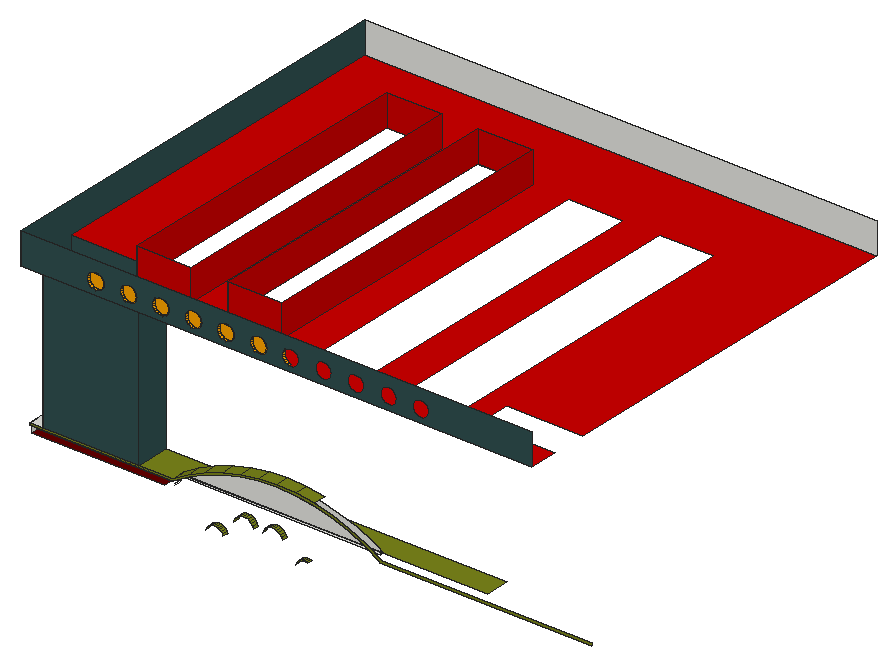
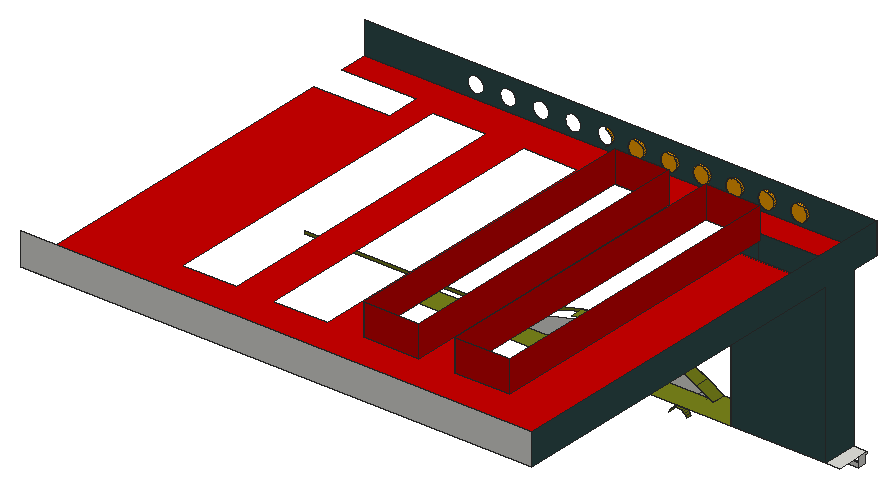
# SketchUp Ruby script. Lengths in inches.
U = 1.inch
M = Sketchup.active_model
def pt(a) = Geom::Point3d.new(a.map { |v| v * U })
def face(e, loops, mat)
  f = e.add_face(loops[0].map { |a| pt(a) })
  loops[1..].each { |l| e.add_face(l.map { |a| pt(a) }).erase! }
  f.material = f.back_material = mat if mat
  f
end
# faces: each face lists its corners as indices into pts; further lists are holes
def faces(e, pts, list, mat = nil) = list.each { |f| face(e, (f[0].is_a?(Array) ? f : [f]).map { |l| l.map { |i| pts[i] } }, mat) }
# xy, xz, yz: faces in a plane at the given z, y or x. An outline is a flat list of corners, or four numbers for a rectangle; further outlines are holes
def ring(l) = l.size == 4 ? [[l[0], l[1]], [l[2], l[1]], [l[2], l[3]], [l[0], l[3]]] : l.each_slice(2).to_a
def flat(e, list, mat, &to3) = list.each { |f| face(e, (f[0].is_a?(Array) ? f : [f]).map { |l| ring(l).map { |u, v| to3.(u, v) } }, mat) }
def xy(e, z, list, mat = nil) = flat(e, list, mat) { |x, y| [x, y, z] }
def xz(e, y, list, mat = nil) = flat(e, list, mat) { |x, z| [x, y, z] }
def yz(e, x, list, mat = nil) = flat(e, list, mat) { |y, z| [x, y, z] }
def lines(e, pts, list) = list.each { |a, b| e.add_line(pt(pts[a]), pt(pts[b])) }
# prism: a flat outline (further loops are holes) pulled along v
def prism(e, loops, v, mat = nil)
  f = face(e, loops, mat); d = Geom::Vector3d.new(v.map { |x| x * U })
  f.pushpull(f.normal.samedirection?(d) ? d.length : -d.length)
end
def box(e, o, s, mat = nil) = prism(e, [[o, [o[0] + s[0], o[1], o[2]], [o[0] + s[0], o[1] + s[1], o[2]], [o[0], o[1] + s[1], o[2]]]], [0, 0, s[2]], mat)
def at(x, y, z, deg = 0) = Geom::Transformation.translation(pt([x, y, z])) * Geom::Transformation.rotation(ORIGIN, Z_AXIS, deg.degrees)
def axes(o, x, y, z) = Geom::Transformation.new([*x, 0, *y, 0, *z, 0, *pt(o).to_a, 1])
def part(name) = M.definitions.add(name)
# library, detail: a bought-in or finely detailed component or shape, given as its bounding box
def library(name, o, s) = part(name).tap { |d| box(d.entities, o, s) }
def detail(e, o, s) = box(e.add_group.entities, o, s)
def put(e, d, t, mat = nil) = e.add_instance(d, t).tap { |i| i.material = mat if mat }
def group(e, t, mat = nil) = e.add_group.tap { |g| g.transformation = t; g.material = mat if mat }.entities
root = M.entities
M.materials.add("[0020_Red]1").color = [204, 0, 0]
M.materials.add("[0022_Maroon]").color = [99, 0, 0]
M.materials.add("[0038_Orange]1").color = [255, 165, 0]
M.materials.add("[0057_DarkKhaki]").color = [122, 132, 27]
M.materials.add("[0078_DarkSlateGray]").color = [47, 79, 79]
xy(root,296.97,[[7,639.11,57.84,642.11]],"[0022_Maroon]")
xy(root,299.95,[[7,638.11,7.79,639.11]])
xy(root,299.95,[[7.79,638.11,61.62,639.11]],"[0057_DarkKhaki]")
xy(root,300.6875,[[64.08,640.93,138.48,642.11]])
xy(root,300.74,[[7,638.11,12.25,651.24],[12.25,638.11,48.5,651.24],[64.16,642.11,138.39,642.18]])
xy(root,300.74,[[48.5,638.11,61.4,638.11,61.4,642.11,64.16,642.11,64.16,642.18,138.39,642.18,138.39,642.11,178.3125,642.11,178.3125,651.24,48.5,651.24]],"[0057_DarkKhaki]")
xy(root,360.74,[[45.02,641.59,48.5,651.24]])
xy(root,360.74,[[[12.25,627.18,12.25,638.11,48.5,638.11,48.5,641.59,65.77,641.59,65.77,760.78,45.02,760.78,45.02,651.24,12.25,651.24,12.25,791.05,207,791.05,207,651.24,178.3125,651.24,178.3125,638.05,207,638.05,207,627.18],[79.64,641.59,100.39,760.78],[114.27,641.59,135.02,760.78],[148.89,641.59,169.64,760.78]]],"[0020_Red]1")
xz(root,627.18,[[[12.25,360.74,207,372.74],[164.76,362.59,163.97,362.69,163.23,363,162.59,363.48,162.11,364.12,161.8,364.86,161.7,365.65,161.8,366.44,162.11,367.18,162.59,367.82,163.23,368.3,163.97,368.61,164.76,368.71,165.55,368.61,166.29,368.3,166.92,367.82,167.41,367.18,167.72,366.44,167.82,365.65,167.72,364.86,167.41,364.12,166.92,363.48,166.29,363,165.55,362.69],[152.38,362.59,151.59,362.69,150.85,363,150.22,363.48,149.73,364.12,149.43,364.86,149.32,365.65,149.43,366.44,149.73,367.18,150.22,367.82,150.85,368.3,151.59,368.61,152.38,368.71,153.18,368.61,153.91,368.3,154.55,367.82,155.04,367.18,155.34,366.44,155.45,365.65,155.34,364.86,155.04,364.12,154.55,363.48,153.91,363,153.18,362.69],[140.01,362.59,139.22,362.69,138.48,363,137.84,363.48,137.36,364.12,137.05,364.86,136.95,365.65,137.05,366.44,137.36,367.18,137.84,367.82,138.48,368.3,139.22,368.61,140.01,368.71,140.8,368.61,141.54,368.3,142.17,367.82,142.66,367.18,142.97,366.44,143.07,365.65,142.97,364.86,142.66,364.12,142.17,363.48,141.54,363,140.8,362.69],[127.63,362.59,126.84,362.69,126.1,363,125.47,363.48,124.98,364.12,124.68,364.86,124.57,365.65,124.68,366.44,124.98,367.18,125.47,367.82,126.1,368.3,126.84,368.61,127.63,368.71,128.43,368.61,129.16,368.3,129.8,367.82,130.29,367.18,130.59,366.44,130.7,365.65,130.59,364.86,130.29,364.12,129.8,363.48,129.16,363,128.43,362.69],[115.26,362.59,114.47,362.69,113.73,363,113.09,363.48,112.61,364.12,112.3,364.86,112.2,365.65,112.3,366.44,112.61,367.18,113.09,367.82,113.73,368.3,114.47,368.61,115.26,368.71,116.05,368.61,116.79,368.3,117.42,367.82,117.91,367.18,118.22,366.44,118.32,365.65,118.22,364.86,117.91,364.12,117.42,363.48,116.79,363,116.05,362.69],[102.88,362.59,102.09,362.69,101.35,363,100.72,363.48,100.23,364.12,99.93,364.86,99.82,365.65,99.93,366.44,100.23,367.18,100.72,367.82,101.35,368.3,102.09,368.61,102.88,368.71,103.68,368.61,104.41,368.3,105.05,367.82,105.54,367.18,105.84,366.44,105.95,365.65,105.84,364.86,105.54,364.12,105.05,363.48,104.41,363,103.68,362.69],[90.51,362.59,89.72,362.69,88.98,363,88.34,363.48,87.86,364.12,87.55,364.86,87.45,365.65,87.55,366.44,87.86,367.18,88.34,367.82,88.98,368.3,89.72,368.61,90.51,368.71,91.3,368.61,92.04,368.3,92.67,367.82,93.16,367.18,93.47,366.44,93.57,365.65,93.47,364.86,93.16,364.12,92.67,363.48,92.04,363,91.3,362.69],[78.13,362.59,77.34,362.69,76.6,363,75.97,363.48,75.48,364.12,75.18,364.86,75.07,365.65,75.18,366.44,75.48,367.18,75.97,367.82,76.6,368.3,77.34,368.61,78.13,368.71,78.93,368.61,79.66,368.3,80.3,367.82,80.79,367.18,81.09,366.44,81.2,365.65,81.09,364.86,80.79,364.12,80.3,363.48,79.66,363,78.93,362.69],[65.76,362.59,64.97,362.69,64.23,363,63.59,363.48,63.11,364.12,62.8,364.86,62.7,365.65,62.8,366.44,63.11,367.18,63.59,367.82,64.23,368.3,64.97,368.61,65.76,368.71,66.55,368.61,67.29,368.3,67.92,367.82,68.41,367.18,68.72,366.44,68.82,365.65,68.72,364.86,68.41,364.12,67.92,363.48,67.29,363,66.55,362.69],[53.38,362.59,52.59,362.69,51.85,363,51.22,363.48,50.73,364.12,50.43,364.86,50.32,365.65,50.43,366.44,50.73,367.18,51.22,367.82,51.85,368.3,52.59,368.61,53.38,368.71,54.18,368.61,54.91,368.3,55.55,367.82,56.04,367.18,56.34,366.44,56.45,365.65,56.34,364.86,56.04,364.12,55.55,363.48,54.91,363,54.18,362.69],[41.01,362.59,40.22,362.69,39.48,363,38.84,363.48,38.36,364.12,38.05,364.86,37.95,365.65,38.05,366.44,38.36,367.18,38.84,367.82,39.48,368.3,40.22,368.61,41.01,368.71,41.8,368.61,42.54,368.3,43.17,367.82,43.66,367.18,43.97,366.44,44.07,365.65,43.97,364.86,43.66,364.12,43.17,363.48,42.54,363,41.8,362.69]]],"[0078_DarkSlateGray]")
xz(root,628.18,[[41.01,362.59,41.8,362.69,42.54,363,43.17,363.48,43.66,364.12,43.97,364.86,44.07,365.65,43.97,366.44,43.66,367.18,43.17,367.82,42.54,368.3,41.8,368.61,41.01,368.71,40.22,368.61,39.48,368.3,38.84,367.82,38.36,367.18,38.05,366.44,37.95,365.65,38.05,364.86,38.36,364.12,38.84,363.48,39.48,363,40.22,362.69],[53.38,362.59,54.18,362.69,54.91,363,55.55,363.48,56.04,364.12,56.34,364.86,56.45,365.65,56.34,366.44,56.04,367.18,55.55,367.82,54.91,368.3,54.18,368.61,53.38,368.71,52.59,368.61,51.85,368.3,51.22,367.82,50.73,367.18,50.43,366.44,50.32,365.65,50.43,364.86,50.73,364.12,51.22,363.48,51.85,363,52.59,362.69],[65.76,362.59,66.55,362.69,67.29,363,67.92,363.48,68.41,364.12,68.72,364.86,68.82,365.65,68.72,366.44,68.41,367.18,67.92,367.82,67.29,368.3,66.55,368.61,65.76,368.71,64.97,368.61,64.23,368.3,63.59,367.82,63.11,367.18,62.8,366.44,62.7,365.65,62.8,364.86,63.11,364.12,63.59,363.48,64.23,363,64.97,362.69],[78.13,362.59,78.93,362.69,79.66,363,80.3,363.48,80.79,364.12,81.09,364.86,81.2,365.65,81.09,366.44,80.79,367.18,80.3,367.82,79.66,368.3,78.93,368.61,78.13,368.71,77.34,368.61,76.6,368.3,75.97,367.82,75.48,367.18,75.18,366.44,75.07,365.65,75.18,364.86,75.48,364.12,75.97,363.48,76.6,363,77.34,362.69],[90.51,362.59,91.3,362.69,92.04,363,92.67,363.48,93.16,364.12,93.47,364.86,93.57,365.65,93.47,366.44,93.16,367.18,92.67,367.82,92.04,368.3,91.3,368.61,90.51,368.71,89.72,368.61,88.98,368.3,88.34,367.82,87.86,367.18,87.55,366.44,87.45,365.65,87.55,364.86,87.86,364.12,88.34,363.48,88.98,363,89.72,362.69],
  [102.88,362.59,103.68,362.69,104.41,363,105.05,363.48,105.54,364.12,105.84,364.86,105.95,365.65,105.84,366.44,105.54,367.18,105.05,367.82,104.41,368.3,103.68,368.61,102.88,368.71,102.09,368.61,101.35,368.3,100.72,367.82,100.23,367.18,99.93,366.44,99.82,365.65,99.93,364.86,100.23,364.12,100.72,363.48,101.35,363,102.09,362.69]],"[0038_Orange]1")
xz(root,638.11,[[140.36,299.9,221.0625,299.9,221.0625,300.74,141.15,300.74,135.09,304.29,128.71,307.25,122.08,309.58,115.25,311.26,108.3,312.27,101.28,312.61,94.26,312.27,87.3,311.26,80.47,309.58,73.84,307.25,67.46,304.29,61.4,300.74,7,300.74,7,299.95,61.62,299.95,67.83,303.6,74.14,306.52,80.7,308.82,87.45,310.48,94.33,311.49,101.28,311.82,108.22,311.49,115.1,310.48,121.85,308.82,128.42,306.52,134.72,303.6,140.36,300.29]],"[0057_DarkKhaki]")
xz(root,638.11,[[12.25,300.74,48.5,360.74]],"[0078_DarkSlateGray]")
xz(root,641.59,[[45.02,360.74,65.77,372.74],[79.64,360.74,100.39,372.74]],"[0020_Red]1")
xz(root,642.11,[[7,296.97,57.84,296.97,57.84,298.09,61.4,298.09,61.4,298.66,7,298.66],[61.4,300.61,64.16,300.6875],[64.16,300.67,138.39,300.6875],[61.4,300.6875,64.08,300.6875,64.16,300.74,61.4,300.74],[64.08,300.6875,64.16,300.74,64.16,300.6875],
  [64.16,300.6875,138.39,300.74]])
xz(root,642.18,[[64.16,300.74,138.39,300.74,136.01,302.13,134.44,303.06,128.1875,305.96,121.68,308.24,114.99,309.89,108.16,310.88,101.28,311.21,94.39,310.88,87.57,309.89,80.87,308.24,74.37,305.96,68.11,303.06,66.54,302.13]])
xz(root,651.24,[[12.25,300.74,48.5,360.74]],"[0078_DarkSlateGray]")
xz(root,760.78,[[45.02,360.74,65.77,372.74],[79.64,360.74,100.39,372.74]],"[0020_Red]1")
xz(root,791.05,[[12.25,360.74,207,372.74]])
yz(root,7,[[639.11,296.97,639.11,299.95,638.11,299.95,638.11,300.74,642.11,300.74,642.11,296.97]])
yz(root,12.25,[[638.11,300.74,638.11,360.74,627.18,360.74,627.18,372.74,791.05,372.74,791.05,360.74,651.24,360.74,651.24,300.74]],"[0078_DarkSlateGray]")
yz(root,45.02,[[641.59,360.74,760.78,372.74]],"[0020_Red]1")
yz(root,48.5,[[638.11,300.74,651.24,360.74]],"[0078_DarkSlateGray]")
yz(root,61.4,[[642.11,300.61,643.36,300.6875],[642.11,300.6875,643.36,300.74]])
yz(root,65.77,[[641.59,360.74,760.78,372.74]],"[0020_Red]1")
yz(root,79.64,[[641.59,360.74,760.78,372.74]],"[0020_Red]1")
yz(root,100.39,[[641.59,360.74,760.78,372.74]],"[0020_Red]1")
p = [[75.24,639.11,289.31],[74.95,639.11,288.64],[74.95,637.11,288.64],[75.24,637.11,289.31],[81.57,639.11,288.64],[81.27,639.11,289.31],
  [81.27,637.11,289.31],[81.57,637.11,288.64],[109.37,639.11,289.31],[109.07,639.11,288.64],[109.07,637.11,288.64],[109.37,637.11,289.31],
  [75.67,639.11,289.9],[75.67,637.11,289.9],[80.85,639.11,289.9],[80.85,637.11,289.9],[109.8,639.11,289.9],[109.8,637.11,289.9],
  [76.21,639.11,290.38],[76.21,637.11,290.38],[80.31,639.11,290.38],[80.31,637.11,290.38],[110.34,639.11,290.38],[110.34,637.11,290.38],
  [76.84,639.11,290.75],[76.84,637.11,290.75],[79.67,639.11,290.75],[79.67,637.11,290.75],[110.97,639.11,290.75],[110.97,637.11,290.75],
  [77.54,639.11,290.97],[77.54,637.11,290.97],[78.98,639.11,290.97],[78.98,637.11,290.97],[111.66,639.11,290.97],[111.66,637.11,290.97],
  [113.8,639.11,290.75],[113.11,639.11,290.97],[113.11,637.11,290.97],[113.8,637.11,290.75],[78.26,639.11,291.05],[78.26,637.11,291.05],
  [112.38,639.11,291.05],[112.38,637.11,291.05],[86.01,639.11,295.99],[85.73,639.11,295.18],[85.73,637.11,295.18],[86.01,637.11,295.99],
  [93.17,639.11,295.18],[92.89,639.11,295.99],[92.89,637.11,295.99],[93.17,637.11,295.18],[96.95,639.11,295.99],[96.67,639.11,295.18],
  [96.67,637.11,295.18],[96.95,637.11,295.99],[104.11,639.11,295.18],[103.83,639.11,295.99],[103.83,637.11,295.99],[104.11,637.11,295.18],
  [86.46,639.11,296.72],[86.46,637.11,296.72],[92.44,639.11,296.72],[92.44,637.11,296.72],[97.4,639.11,296.72],[97.4,637.11,296.72],
  [103.38,639.11,296.72],[103.38,637.11,296.72],[87.0625,639.11,297.33],[87.0625,637.11,297.33],[91.84,639.11,297.33],[91.84,637.11,297.33],
  [98,639.11,297.33],[98,637.11,297.33],[102.78,639.11,297.33],[102.78,637.11,297.33],[87.79,639.11,297.79],[87.79,637.11,297.79],
  [91.12,639.11,297.79],[91.12,637.11,297.79],[98.73,639.11,297.79],[98.73,637.11,297.79],[102.05,639.11,297.79],[102.05,637.11,297.79],
  [88.6,639.11,298.08],[88.6,637.11,298.08],[90.31,639.11,298.08],[90.31,637.11,298.08],[99.54,639.11,298.08],[99.54,637.11,298.08],
  [101.24,639.11,298.08],[101.24,637.11,298.08],[89.45,639.11,298.18],[89.45,637.11,298.18],[100.39,639.11,298.18],[100.39,637.11,298.18],
  [61.62,639.11,299.95],[67.83,639.11,303.6],[67.83,638.11,303.6],[61.62,638.11,299.95],[61.4,642.11,300.74],[61.4,638.11,300.74],
  [67.46,638.11,304.29],[67.46,643.36,304.29],[61.4,643.36,300.74],[74.14,639.11,306.52],[74.14,638.11,306.52],[73.84,638.11,307.25],
  [73.84,643.36,307.25],[80.7,639.11,308.82],[80.7,638.11,308.82],[80.47,638.11,309.58],[80.47,643.36,309.58],[87.45,639.11,310.48],
  [87.45,638.11,310.48],[87.3,638.11,311.26],[87.3,643.36,311.26],[94.33,639.11,311.49],[94.33,638.11,311.49],[108.22,639.11,311.49],
  [115.1,639.11,310.48],[115.1,638.11,310.48],[108.22,638.11,311.49],[94.26,638.11,312.27],[94.26,643.36,312.27],[108.3,643.36,312.27],
  [108.3,638.11,312.27],[115.25,638.11,311.26],[115.25,643.36,311.26],[101.28,639.11,311.82],[101.28,638.11,311.82],[101.28,638.11,312.61],
  [101.28,643.36,312.61],[40.22,627.18,362.69],[41.01,627.18,362.59],[41.01,628.18,362.59],[40.22,628.18,362.69],[41.8,627.18,362.69],
  [41.8,628.18,362.69],[52.59,627.18,362.69],[53.38,627.18,362.59],[53.38,628.18,362.59],[52.59,628.18,362.69],[54.18,627.18,362.69],
  [54.18,628.18,362.69],[64.97,627.18,362.69],[65.76,627.18,362.59],[65.76,628.18,362.59],[64.97,628.18,362.69],[66.55,627.18,362.69],
  [66.55,628.18,362.69],[77.34,627.18,362.69],[78.13,627.18,362.59],[78.13,628.18,362.59],[77.34,628.18,362.69],[78.93,627.18,362.69],
  [78.93,628.18,362.69],[89.72,627.18,362.69],[90.51,627.18,362.59],[90.51,628.18,362.59],[89.72,628.18,362.69],[91.3,627.18,362.69],
  [91.3,628.18,362.69],[102.09,627.18,362.69],[102.88,627.18,362.59],[102.88,628.18,362.59],[102.09,628.18,362.69],[103.68,627.18,362.69],
  [103.68,628.18,362.69],[39.48,627.18,363],[39.48,628.18,363],[42.54,627.18,363],[42.54,628.18,363],[51.85,627.18,363],
  [51.85,628.18,363],[54.91,627.18,363],[54.91,628.18,363],[64.23,627.18,363],[64.23,628.18,363],[67.29,627.18,363],
  [67.29,628.18,363],[76.6,627.18,363],[76.6,628.18,363],[79.66,627.18,363],[79.66,628.18,363],[88.98,627.18,363],
  [88.98,628.18,363],[92.04,627.18,363],[92.04,628.18,363],[101.35,627.18,363],[101.35,628.18,363],[104.41,627.18,363],
  [104.41,628.18,363],[113.73,627.18,363],[114.47,627.18,362.69],[114.47,628.18,362.69],[113.73,628.18,363],[38.84,627.18,363.48],
  [38.84,628.18,363.48],[43.17,627.18,363.48],[43.17,628.18,363.48],[51.22,627.18,363.48],[51.22,628.18,363.48],[55.55,627.18,363.48],
  [55.55,628.18,363.48],[63.59,627.18,363.48],[63.59,628.18,363.48],[67.92,627.18,363.48],[67.92,628.18,363.48],[75.97,627.18,363.48],
  [75.97,628.18,363.48],[80.3,627.18,363.48],[80.3,628.18,363.48],[88.34,627.18,363.48],[88.34,628.18,363.48],[92.67,627.18,363.48],
  [92.67,628.18,363.48],[100.72,627.18,363.48],[100.72,628.18,363.48],[105.05,627.18,363.48],[105.05,628.18,363.48],[113.09,627.18,363.48],
  [113.09,628.18,363.48],[38.36,627.18,364.12],[38.36,628.18,364.12],[43.66,627.18,364.12],[43.66,628.18,364.12],[50.73,627.18,364.12],
  [50.73,628.18,364.12],[56.04,627.18,364.12],[56.04,628.18,364.12],[63.11,627.18,364.12],[63.11,628.18,364.12],[68.41,627.18,364.12],
  [68.41,628.18,364.12],[75.48,627.18,364.12],[75.48,628.18,364.12],[80.79,627.18,364.12],[80.79,628.18,364.12],[87.86,627.18,364.12],
  [87.86,628.18,364.12],[93.16,627.18,364.12],[93.16,628.18,364.12],[100.23,627.18,364.12],[100.23,628.18,364.12],[105.54,627.18,364.12],
  [105.54,628.18,364.12],[112.61,627.18,364.12],[112.61,628.18,364.12],[38.05,627.18,364.86],[38.05,628.18,364.86],[43.97,627.18,364.86],
  [43.97,628.18,364.86],[50.43,627.18,364.86],[50.43,628.18,364.86],[56.34,627.18,364.86],[56.34,628.18,364.86],[62.8,627.18,364.86],
  [62.8,628.18,364.86],[68.72,627.18,364.86],[68.72,628.18,364.86],[75.18,627.18,364.86],[75.18,628.18,364.86],[81.09,627.18,364.86],
  [81.09,628.18,364.86],[87.55,627.18,364.86],[87.55,628.18,364.86],[93.47,627.18,364.86],[93.47,628.18,364.86],[99.93,627.18,364.86],
  [99.93,628.18,364.86],[105.84,627.18,364.86],[105.84,628.18,364.86],[112.3,627.18,364.86],[112.3,628.18,364.86],[37.95,627.18,365.65],
  [37.95,628.18,365.65],[44.07,627.18,365.65],[44.07,628.18,365.65],[50.32,627.18,365.65],[50.32,628.18,365.65],[56.45,627.18,365.65],
  [56.45,628.18,365.65],[62.7,627.18,365.65],[62.7,628.18,365.65],[68.82,627.18,365.65],[68.82,628.18,365.65],[75.07,627.18,365.65],
  [75.07,628.18,365.65],[81.2,627.18,365.65],[81.2,628.18,365.65],[87.45,627.18,365.65],[87.45,628.18,365.65],[93.57,627.18,365.65],
  [93.57,628.18,365.65],[99.82,627.18,365.65],[99.82,628.18,365.65],[105.95,627.18,365.65],[105.95,628.18,365.65],[112.2,627.18,365.65],
  [112.2,628.18,365.65],[38.05,627.18,366.44],[38.05,628.18,366.44],[43.97,627.18,366.44],[43.97,628.18,366.44],[50.43,627.18,366.44],
  [50.43,628.18,366.44],[56.34,627.18,366.44],[56.34,628.18,366.44],[62.8,627.18,366.44],[62.8,628.18,366.44],[68.72,627.18,366.44],
  [68.72,628.18,366.44],[75.18,627.18,366.44],[75.18,628.18,366.44],[81.09,627.18,366.44],[81.09,628.18,366.44],[87.55,627.18,366.44],
  [87.55,628.18,366.44],[93.47,627.18,366.44],[93.47,628.18,366.44],[99.93,627.18,366.44],[99.93,628.18,366.44],[105.84,627.18,366.44],
  [105.84,628.18,366.44],[112.3,627.18,366.44],[112.3,628.18,366.44],[38.36,627.18,367.18],[38.36,628.18,367.18],[43.66,627.18,367.18],
  [43.66,628.18,367.18],[50.73,627.18,367.18],[50.73,628.18,367.18],[56.04,627.18,367.18],[56.04,628.18,367.18],[63.11,627.18,367.18],
  [63.11,628.18,367.18],[68.41,627.18,367.18],[68.41,628.18,367.18],[75.48,627.18,367.18],[75.48,628.18,367.18],[80.79,627.18,367.18],
  [80.79,628.18,367.18],[87.86,627.18,367.18],[87.86,628.18,367.18],[93.16,627.18,367.18],[93.16,628.18,367.18],[100.23,627.18,367.18],
  [100.23,628.18,367.18],[105.54,627.18,367.18],[105.54,628.18,367.18],[112.61,627.18,367.18],[112.61,628.18,367.18],[38.84,627.18,367.82],
  [38.84,628.18,367.82],[43.17,627.18,367.82],[43.17,628.18,367.82],[51.22,627.18,367.82],[51.22,628.18,367.82],[55.55,627.18,367.82],
  [55.55,628.18,367.82],[63.59,627.18,367.82],[63.59,628.18,367.82],[67.92,627.18,367.82],[67.92,628.18,367.82],[75.97,627.18,367.82],
  [75.97,628.18,367.82],[80.3,627.18,367.82],[80.3,628.18,367.82],[88.34,627.18,367.82],[88.34,628.18,367.82],[92.67,627.18,367.82],
  [92.67,628.18,367.82],[100.72,627.18,367.82],[100.72,628.18,367.82],[105.05,627.18,367.82],[105.05,628.18,367.82],[113.09,627.18,367.82],
  [113.09,628.18,367.82],[39.48,627.18,368.3],[39.48,628.18,368.3],[42.54,627.18,368.3],[42.54,628.18,368.3],[51.85,627.18,368.3],
  [51.85,628.18,368.3],[54.91,627.18,368.3],[54.91,628.18,368.3],[64.23,627.18,368.3],[64.23,628.18,368.3],[67.29,627.18,368.3],
  [67.29,628.18,368.3],[76.6,627.18,368.3],[76.6,628.18,368.3],[79.66,627.18,368.3],[79.66,628.18,368.3],[88.98,627.18,368.3],
  [88.98,628.18,368.3],[92.04,627.18,368.3],[92.04,628.18,368.3],[101.35,627.18,368.3],[101.35,628.18,368.3],[104.41,627.18,368.3],
  [104.41,628.18,368.3],[113.73,627.18,368.3],[113.73,628.18,368.3],[40.22,627.18,368.61],[40.22,628.18,368.61],[41.8,627.18,368.61],
  [41.8,628.18,368.61],[52.59,627.18,368.61],[52.59,628.18,368.61],[54.18,627.18,368.61],[54.18,628.18,368.61],[64.97,627.18,368.61],
  [64.97,628.18,368.61],[66.55,627.18,368.61],[66.55,628.18,368.61],[77.34,627.18,368.61],[77.34,628.18,368.61],[78.93,627.18,368.61],
  [78.93,628.18,368.61],[89.72,627.18,368.61],[89.72,628.18,368.61],[91.3,627.18,368.61],[91.3,628.18,368.61],[102.09,627.18,368.61],
  [102.09,628.18,368.61],[103.68,627.18,368.61],[103.68,628.18,368.61],[114.47,627.18,368.61],[114.47,628.18,368.61],[41.01,627.18,368.71],
  [41.01,628.18,368.71],[53.38,627.18,368.71],[53.38,628.18,368.71],[65.76,627.18,368.71],[65.76,628.18,368.71],[78.13,627.18,368.71],
  [78.13,628.18,368.71],[90.51,627.18,368.71],[90.51,628.18,368.71],[102.88,627.18,368.71],[102.88,628.18,368.71],[66.54,643.36,302.13],
  [66.54,642.18,302.13],[64.16,642.18,300.74],[64.16,643.36,300.74],[61.4,642.11,298.66],[61.4,639.11,298.66],[61.4,642.11,300.61],
  [61.4,639.11,300.61],[61.4,642.11,300.6875],[61.4,639.11,300.6875],[61.4,642.11,298.09],[61.4,639.11,298.09]]
faces(root,p,[[0,1,2,3],[4,5,6,7],[8,9,10,11],[12,0,3,13],[5,14,15,6],[16,8,11,17],[18,12,13,19],[14,20,21,15],
  [22,16,17,23],[24,18,19,25],[20,26,27,21],[28,22,23,29],[30,24,25,31],[26,32,33,27],[34,28,29,35],[36,37,38,39],
  [40,30,31,41],[32,40,41,33],[42,34,35,43],[37,42,43,38],[44,45,46,47],[48,49,50,51],[52,53,54,55],[56,57,58,59],
  [60,44,47,61],[49,62,63,50],[64,52,55,65],[57,66,67,58],[68,60,61,69],[62,70,71,63],[72,64,65,73],[66,74,75,67],
  [76,68,69,77],[70,78,79,71],[80,72,73,81],[74,82,83,75],[84,76,77,85],[78,86,87,79],[88,80,81,89],[82,90,91,83],
  [92,84,85,93],[86,92,93,87],[94,88,89,95],[90,94,95,91],[96,97,98,99],[100,101,102,103,104],[97,105,106,98],[103,102,107,108],
  [105,109,110,106],[108,107,111,112],[109,113,114,110],[112,111,115,116],[113,117,118,114],[119,120,121,122],[116,115,123,124],[125,126,127,128],
  [117,129,130,118],[129,119,122,130],[124,123,131,132],[132,131,126,125]],"[0057_DarkKhaki]")
faces(root,p,[[133,134,135,136],[134,137,138,135],[139,140,141,142],[140,143,144,141],[145,146,147,148],[146,149,150,147],[151,152,153,154],[152,155,156,153],
  [157,158,159,160],[158,161,162,159],[163,164,165,166],[164,167,168,165],[169,133,136,170],[137,171,172,138],[173,139,142,174],[143,175,176,144],
  [177,145,148,178],[149,179,180,150],[181,151,154,182],[155,183,184,156],[185,157,160,186],[161,187,188,162],[189,163,166,190],[167,191,192,168],
  [193,194,195,196],[197,169,170,198],[171,199,200,172],[201,173,174,202],[175,203,204,176],[205,177,178,206],[179,207,208,180],[209,181,182,210],
  [183,211,212,184],[213,185,186,214],[187,215,216,188],[217,189,190,218],[191,219,220,192],[221,193,196,222],[223,197,198,224],[199,225,226,200],
  [227,201,202,228],[203,229,230,204],[231,205,206,232],[207,233,234,208],[235,209,210,236],[211,237,238,212],[239,213,214,240],[215,241,242,216],
  [243,217,218,244],[219,245,246,220],[247,221,222,248],[249,223,224,250],[225,251,252,226],[253,227,228,254],[229,255,256,230],[257,231,232,258],
  [233,259,260,234],[261,235,236,262],[237,263,264,238],[265,239,240,266],[241,267,268,242],[269,243,244,270],[245,271,272,246],[273,247,248,274],
  [275,249,250,276],[251,277,278,252],[279,253,254,280],[255,281,282,256],[283,257,258,284],[259,285,286,260],[287,261,262,288],[263,289,290,264],
  [291,265,266,292],[267,293,294,268],[295,269,270,296],[271,297,298,272],[299,273,274,300],[301,275,276,302],[277,303,304,278],[305,279,280,306],
  [281,307,308,282],[309,283,284,310],[285,311,312,286],[313,287,288,314],[289,315,316,290],[317,291,292,318],[293,319,320,294],[321,295,296,322],
  [297,323,324,298],[325,299,300,326],[327,301,302,328],[303,329,330,304],[331,305,306,332],[307,333,334,308],[335,309,310,336],[311,337,338,312],
  [339,313,314,340],[315,341,342,316],[343,317,318,344],[319,345,346,320],[347,321,322,348],[323,349,350,324],[351,325,326,352],[353,327,328,354],
  [329,355,356,330],[357,331,332,358],[333,359,360,334],[361,335,336,362],[337,363,364,338],[365,339,340,366],[341,367,368,342],[369,343,344,370],
  [345,371,372,346],[373,347,348,374],[349,375,376,350],[377,351,352,378],[379,353,354,380],[355,381,382,356],[383,357,358,384],[359,385,386,360],
  [387,361,362,388],[363,389,390,364],[391,365,366,392],[367,393,394,368],[395,369,370,396],[371,397,398,372],[399,373,374,400],[375,401,402,376],
  [403,377,378,404],[405,379,380,406],[381,407,408,382],[409,383,384,410],[385,411,412,386],[413,387,388,414],[389,415,416,390],[417,391,392,418],
  [393,419,420,394],[421,395,396,422],[397,423,424,398],[425,399,400,426],[401,427,428,402],[429,403,404,430],[431,405,406,432],[407,431,432,408],
  [433,409,410,434],[411,433,434,412],[435,413,414,436],[415,435,436,416],[437,417,418,438],[419,437,438,420],[439,421,422,440],[423,439,440,424],
  [441,425,426,442],[427,441,442,428]],"[0038_Orange]1")
lines(root,p,[[443,444],[445,446],[447,448],[449,450],[451,452],[453,454]])
